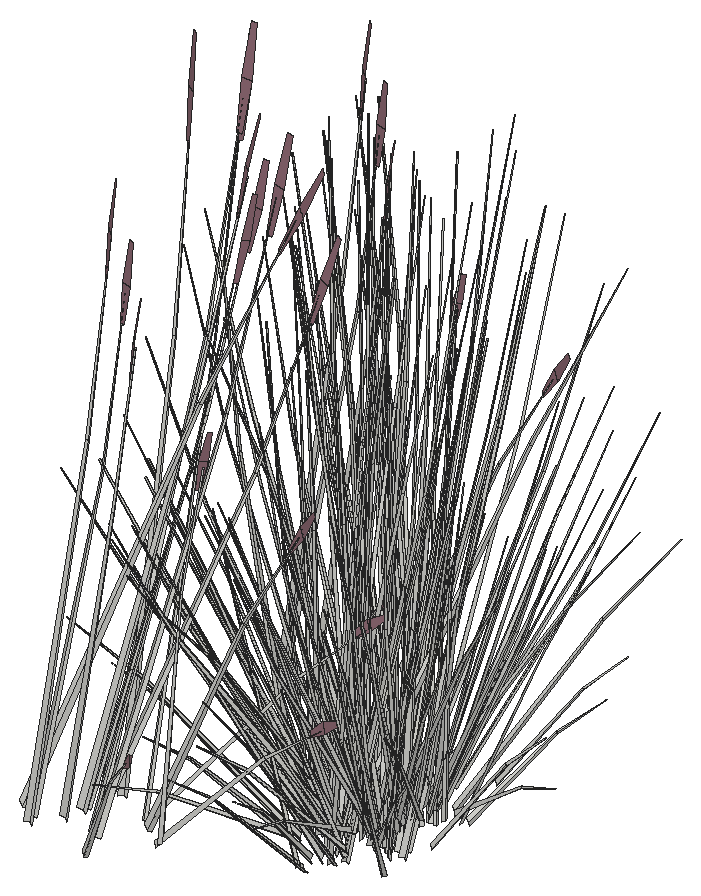
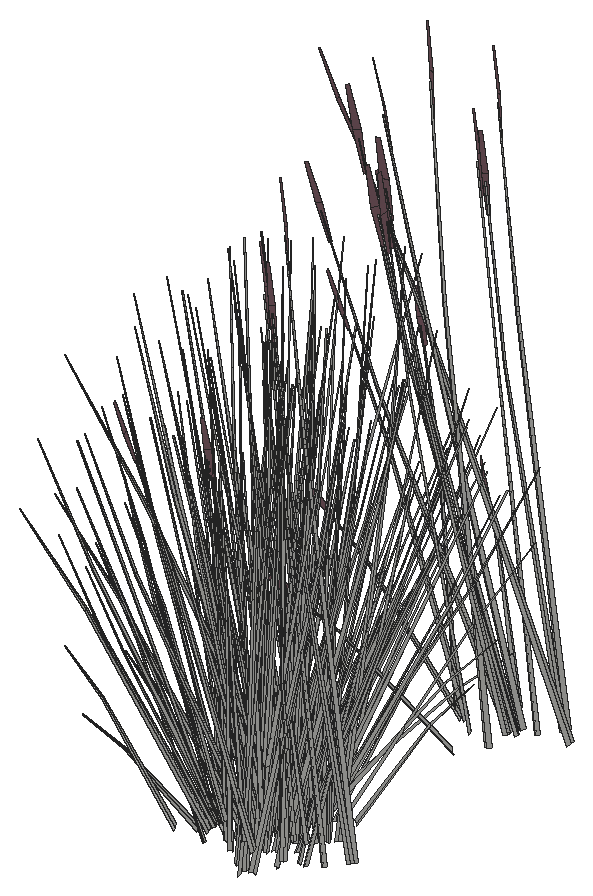
# SketchUp Ruby script. Lengths in inches.
U = 1.inch
M = Sketchup.active_model
def pt(a) = Geom::Point3d.new(a.map { |v| v * U })
def face(e, loops, mat)
  f = e.add_face(loops[0].map { |a| pt(a) })
  loops[1..].each { |l| e.add_face(l.map { |a| pt(a) }).erase! }
  f.material = f.back_material = mat if mat
  f
end
# faces: each face lists its corners as indices into pts; further lists are holes
def faces(e, pts, list, mat = nil) = list.each { |f| face(e, (f[0].is_a?(Array) ? f : [f]).map { |l| l.map { |i| pts[i] } }, mat) }
# xy, xz, yz: faces in a plane at the given z, y or x. An outline is a flat list of corners, or four numbers for a rectangle; further outlines are holes
def ring(l) = l.size == 4 ? [[l[0], l[1]], [l[2], l[1]], [l[2], l[3]], [l[0], l[3]]] : l.each_slice(2).to_a
def flat(e, list, mat, &to3) = list.each { |f| face(e, (f[0].is_a?(Array) ? f : [f]).map { |l| ring(l).map { |u, v| to3.(u, v) } }, mat) }
def xy(e, z, list, mat = nil) = flat(e, list, mat) { |x, y| [x, y, z] }
def xz(e, y, list, mat = nil) = flat(e, list, mat) { |x, z| [x, y, z] }
def yz(e, x, list, mat = nil) = flat(e, list, mat) { |y, z| [x, y, z] }
def lines(e, pts, list) = list.each { |a, b| e.add_line(pt(pts[a]), pt(pts[b])) }
# prism: a flat outline (further loops are holes) pulled along v
def prism(e, loops, v, mat = nil)
  f = face(e, loops, mat); d = Geom::Vector3d.new(v.map { |x| x * U })
  f.pushpull(f.normal.samedirection?(d) ? d.length : -d.length)
end
def box(e, o, s, mat = nil) = prism(e, [[o, [o[0] + s[0], o[1], o[2]], [o[0] + s[0], o[1] + s[1], o[2]], [o[0], o[1] + s[1], o[2]]]], [0, 0, s[2]], mat)
def at(x, y, z, deg = 0) = Geom::Transformation.translation(pt([x, y, z])) * Geom::Transformation.rotation(ORIGIN, Z_AXIS, deg.degrees)
def axes(o, x, y, z) = Geom::Transformation.new([*x, 0, *y, 0, *z, 0, *pt(o).to_a, 1])
def part(name) = M.definitions.add(name)
# library, detail: a bought-in or finely detailed component or shape, given as its bounding box
def library(name, o, s) = part(name).tap { |d| box(d.entities, o, s) }
def detail(e, o, s) = box(e.add_group.entities, o, s)
def put(e, d, t, mat = nil) = e.add_instance(d, t).tap { |i| i.material = mat if mat }
def group(e, t, mat = nil) = e.add_group.tap { |g| g.transformation = t; g.material = mat if mat }.entities
root = M.entities
M.materials.add("LightPink_Translucent").color = [144, 107, 117]
c1 = part("blade")
p = [[2.15,0.21,22],[0,0.17,0],[0.09,0.45,0],[2.18,0.31,22],[2.29,0.31,22],[0.38,0.45,0],
  [2.48,0.24,33],[2.49,0.24,33],[2.48,0.22,33]]
faces(c1.entities,p,[[0,1,2,3],[4,5,2,3],[6,3,4,7],[8,0,3,6]])
c2 = part("seeds")
p = [[0.3,-0.1,1.38],[-0.01,-0.03,1.59],[-0.01,-0.03,0.03],[0.14,-0.07,-0.07],[0.29,-0.03,3],[0.15,0.01,3.11]]
faces(c2.entities,p,[[0,1,2,3],[1,0,4,5]],"LightPink_Translucent")
c3 = part("blade with seeds")
put(c3.entities,c1,at(0,0,0))
put(c3.entities,c2,axes([2.4,0.25,30.99],[1.5799,-0.05474,1.17369],[-0.12525,1.92788,0.29478],[-0.07173,-0.02425,1.56792]))
c4 = part("blade with seeds\#1")
put(c4.entities,c1,at(0,0,0))
put(root,c3,axes([62.45,49.91,44.03],[1.14332,0.25625,-0.30978],[-0.28787,0.90242,0.30978],[0.23049,-0.10406,1.38974]))
put(root,c4,axes([73.33,39.71,40.79],[-0.89213,0.297,-0.46065],[-0.15606,-1.12475,-0.35681],[-0.23962,-0.32232,0.88141]))
put(root,c3,axes([65.59,26.18,44.67],[1.38012,0.49416,-0.29095],[-0.66454,1.04299,-0.50002],[0.04337,0.25608,1.59708]))
put(root,c4,axes([73.69,39.68,41.0625],[-0.77091,-0.6039,-0.64046],[0.54787,-1.05824,0.07729],[-0.27931,-0.36058,0.906]))
put(root,c3,axes([62.65,22.63,44.03],[1.14332,0.25625,-0.30978],[-0.28787,0.90242,0.30978],[0.23049,-0.10406,1.38974]))
put(root,c4,axes([73.97,39.18,41.11],[-0.53874,1.06944,-0.10962],[-0.78019,-0.61612,-0.60845],[-0.2712,-0.30214,0.92453]))
put(root,c3,axes([62.18,49.5,44.02],[1.14694,-0.51783,-0.49651],[0.68554,0.92854,0],[0.26122,-0.11794,1.57504]))
put(root,c3,axes([69.18,27.38,44.02],[0,1.03566,-0.49651],[-1.37109,0,0],[0,0.23588,1.57504]))
put(root,c4,axes([71.58,45.69,41.13],[0.78697,-0.17856,0.31925],[0.2078,1.02074,-0.41216],[-0.22552,0.27417,0.78863]))
put(root,c3,axes([62.38,22.22,44.02],[1.14694,-0.51783,-0.49651],[0.68554,0.92854,0],[0.26122,-0.11794,1.57504]))
put(root,c4,axes([72.98,38.81,38.91],[-0.02894,0.41302,1.28914],[-0.77632,0.42312,-0.27724],[-0.21961,-0.50739,0.55117]))
put(root,c4,axes([71.29,45.23,38.39],[-0.48852,-1.08202,-0.44759],[0.87598,-0.64674,0],[-0.11126,-0.24644,1.41987]))
put(root,c4,axes([73.73,36.55,40.82],[-0.00742,0.151,1.59908],[-0.79509,0.62706,-0.1511],[-0.26143,-0.25182,0.28298]))
put(root,c4,axes([71.56,38.33,39.07],[0.49736,0.38508,1.03545],[-0.66822,0.331,0.76078],[-0.16744,-0.31805,0.22807]))
put(root,c4,axes([74.1875,48.82,38.39],[-0.97703,0,-0.44759],[0,-1.29348,0],[-0.22253,0,1.41987]))
put(root,c4,axes([76.91,43.6,39.57],[0.39398,-0.99907,1.36359],[0.84877,0.97875,0.53923],[-0.50305,0.4384,1.14314]))
put(root,c4,axes([73.3,43.94,38.43],[-0.73437,-0.77871,-0.5621],[0.66591,-0.96736,-0.14753],[-0.18319,-0.31204,1.24074]))
put(root,c3,axes([65.33,28.59,44.18],[1.2866,-0.3514,-0.19198],[0.45209,1.01223,0.00008],[0.14202,-0.03884,1.73897]))
put(root,c4,axes([73.42,38.88,40.65],[-0.13963,-1.00636,-0.31925],[0.79822,-0.26574,0.41216],[-0.2144,-0.28839,0.78863]))
put(root,c4,axes([74.58,45.3,38.57],[-0.88038,-0.56093,-0.40331],[0.4237,-1.16553,0.1941],[-0.20294,0,1.29492]))
put(root,c4,axes([73.9,39.7,41.13],[0.13963,1.00636,0.31925],[-0.79822,0.26574,-0.41216],[-0.2144,-0.28839,0.78863]))
put(root,c4,axes([74.15,44.79,38.98],[-1.11485,0.13472,-0.26229],[-0.06741,-1.40314,-0.45076],[-0.1485,-0.24708,1.43974]))
put(root,c4,axes([74.21,48.27,38.4],[-0.60959,-0.80703,-0.27926],[0.60959,-0.80703,0.27926],[-0.19635,0,1.25283]))
put(root,c4,axes([75.32,45.44,38.98],[-0.46619,1.302,-0.26229],[-0.98396,-0.62692,-0.45076],[-0.24158,0.04092,1.43974]))
put(root,c4,axes([74.93,49.14,38.71],[0,1.44565,0],[-1.09198,0,-0.46523],[-0.24871,0,1.47583]))
put(root,c3,axes([65.35,25.58,44.21],[0.73619,0.86927,-0.44739],[-1.11511,0.61213,0.21531],[0.23824,0.10756,1.43643]))
put(root,c4,axes([71.68,44.97,38.4],[0.24175,-1.0786,-0.27926],[0.85134,0.27158,0.27926],[-0.09817,-0.21744,1.25283]))
put(root,c3,axes([63.54,51.63,44.06],[0.82544,-0.77843,-0.62353],[1.0254,0.70586,-0.16365],[0.33076,-0.19418,1.37633]))
put(root,c3,axes([63.74,24.34,44.06],[0.82544,-0.77843,-0.62353],[1.0254,0.70586,-0.16365],[0.33076,-0.19418,1.37633]))
put(root,c4,axes([73.6,39.01,40.84],[0.89921,-0.28673,0.43274],[0.15606,1.12475,0.35681],[-0.21148,-0.33149,0.89544]))
put(root,c4,axes([73.77,38.79,40.84],[0.4109,-0.79368,0.05797],[0.58514,0.46209,0.45634],[-0.18917,-0.25446,0.69585]))
put(root,c4,axes([74.68,35.98,40.82],[-0.14882,-0.16043,1.57709],[-0.91289,0.20534,-0.24942],[-0.17308,-0.40254,0.12648]))
put(root,c4,axes([74.64,48.02,38.67],[0.82143,1.07538,0.27726],[-0.81279,1.07603,-0.32897],[-0.23327,0.03755,1.48641]))
put(root,c3,axes([67.37,23.65,44.03],[0.28787,0.90242,-0.30978],[-1.14332,0.25625,0.30978],[0.23049,0.10406,1.38974]))
put(root,c3,axes([64.57,25.09,44.67],[1.23732,-0.68758,-0.29095],[0.8228,0.97154,-0.50002],[0.30528,0.09867,1.59708]))
put(root,c4,axes([75.02,44.6,38.77],[0.47355,-1.30265,0.21694],[0.98396,0.62692,0.45076],[-0.22682,0,1.44726]))
put(root,c4,axes([76.35,45.11,38.77],[-1.15773,-0.30643,-0.21121],[0.20181,-1.4529,0.4622],[-0.15988,0.25387,1.41028]))
put(root,c4,axes([74.36,45.02,39.02],[0.06031,1.25545,0.40331],[-1.00118,0.11354,-0.1941],[-0.10147,-0.22475,1.29492]))
put(root,c4,axes([75.09,48.27,38.81],[0.97703,0,0.44759],[0,1.29348,0],[-0.22253,0,1.41987]))
put(root,c4,axes([71.69,40.89,38.72],[-0.97904,-0.72283,0],[0.54599,-1.20931,-0.46523],[0.12435,-0.27543,1.47583]))
put(root,c4,axes([74.72,45.07,38.7],[1.09253,-0.50265,0.41247],[0.37991,1.43622,0.16186],[-0.20075,-0.01755,1.43206]))
put(root,c4,axes([76.07,39.14,41.11],[-0.88471,0.5817,-0.10962],[-0.43476,-1.03242,-0.60845],[-0.11673,-0.43507,0.92453]))
put(root,c4,axes([75.3125,39.1875,40.79],[-0.88873,-0.31321,-0.46065],[0.30463,-1.07385,-0.35681],[-0.08149,-0.43235,0.88141]))
put(root,c4,axes([75.88,45.21,38.57],[-0.82007,0.69452,-0.40331],[-0.57748,-1.05199,0.1941],[-0.10147,0.22475,1.29492]))
put(root,c3,axes([61.44,24.48,43.59],[-1.20625,0.41464,1.28929],[-0.38394,-1.1897,0.50096],[0.74071,0.01979,1.46642]))
put(root,c4,axes([75.5625,38.04,38.36],[0.11725,0.74462,1.27635],[-0.9333,0.11852,0.07306],[-0.14126,-0.52153,0.72629]))
put(root,c4,axes([74.73,36.68,38.61],[-0.62476,0.71677,-0.05849],[-0.57245,-0.78502,-0.26518],[-0.0403,-0.22243,0.87466]))
put(root,c4,axes([72.2,41.51,38.81],[-0.48852,1.08202,0.44759],[-0.87598,-0.64674,0],[0.11126,-0.24644,1.41987]))
put(root,c4,axes([75.58,45.32,39.02],[0.88038,0.56093,0.40331],[-0.4237,1.16553,-0.1941],[-0.20294,0,1.29492]))
put(root,c4,axes([74.82,43.26,38.5625],[-1.1305,0,0],[0,-1.44565,0],[0,0,1.61777]))
put(root,c3,axes([68.0625,49.47,43.49],[-0.18342,-0.08159,1.76342],[-0.47115,-0.9115,-0.26939],[0.31784,-0.24736,0.30037]))
put(root,c4,axes([74.1,43.95,38.7],[0.88667,0.95859,0.41247],[-0.7827,1.13884,0.16186],[-0.08849,-0.2311,1.43206]))
put(root,c3,axes([68.27,22.1875,43.49],[-0.18342,-0.08159,1.76342],[-0.47115,-0.9115,-0.26939],[0.31784,-0.24736,0.30037]))
put(root,c4,axes([72.64,45.61,38.8],[0.971,0.33398,0.15904],[-0.27478,1.22215,0.3163],[-0.00473,-0.21112,1.44604]))
put(root,c4,axes([75.63,39.39,41.0625],[-0.4315,-1.0159,-0.64046],[0.88824,-0.56616,0.07729],[-0.1009,-0.49086,0.906]))
put(root,c4,axes([73.43,46.12,38.01],[0.39117,1.13797,1.16227],[-1.12236,0.3622,0.45161],[0.01867,-0.69878,1.32195]))
put(root,c4,axes([75.69,42.9,38.65],[-0.84094,1.07538,-0.05527],[-0.84146,-1.07603,0],[-0.02937,0.03755,1.58274]))
put(root,c3,axes([67.68,23.26,44.02],[1.14694,0.51783,-0.49651],[-0.68554,0.92854,0],[0.26122,0.11794,1.57504]))
put(root,c4,axes([75.8,39.54,41.13],[-0.27256,0.96081,0.31925],[-0.79518,-0.28024,-0.41216],[-0.07291,-0.38684,0.78863]))
put(root,c3,axes([67.63,30.63,43.49],[0.08928,-0.14952,1.76342],[1.12407,-0.44035,-0.26939],[0.34078,0.22791,0.30037]))
put(root,c4,axes([73.72,43.06,38.93],[-0.87196,-0.22303,0.13053],[0.15136,-1.08968,-0.37274],[0.08953,-0.19831,1.14258]))
put(root,c4,axes([74.95,37.23,37.92],[-0.14833,0.06042,1.5897],[-0.86768,-0.41907,-0.24285],[-0.01248,-0.42273,0.27078]))
put(root,c4,axes([73.95,43.52,39.02],[-0.82007,0.69452,0.40331],[-0.57748,-1.05199,-0.1941],[0.10147,-0.22475,1.29492]))
put(root,c4,axes([75.79,44.94,38.7],[0.20585,-1.46124,0.41247],[1.16261,0.29738,0.16186],[-0.11226,0.21355,1.43206]))
put(root,c3,axes([71.23,53.15,44.26],[-0.75977,-0.66224,-0.06488],[0.83212,-0.6068,-0.29416],[0.23578,-0.04272,0.97024]))
put(root,c3,axes([66.01,25.25,44.06],[1.27479,0.1698,-0.62353],[-0.26901,1.04736,-0.16365],[0.38043,0.12691,1.37633]))
put(root,c3,axes([71.44,25.86,44.26],[-0.75977,-0.66224,-0.06488],[0.83212,-0.6068,-0.29416],[0.23578,-0.04272,0.97024]))
put(root,c4,axes([77.7,47.11,38.4],[-0.85134,0.27158,-0.27926],[-0.24175,-1.0786,0.27926],[-0.09817,0.21744,1.25283]))
put(root,c4,axes([72.28,40.23,38.39],[0.48852,-1.08202,-0.44759],[0.87598,0.64674,0],[0.11126,-0.24644,1.41987]))
put(root,c4,axes([74.01,43.17,38.98],[-0.64866,-1.16728,-0.26229],[0.91655,-0.77622,-0.45076],[0.09308,-0.288,1.43974]))
put(root,c4,axes([72.7,41.91,38.8],[0.25932,1.24233,0.15904],[-0.96507,0.30677,0.3163],[0.14061,-0.1108,1.44604]))
put(root,c4,axes([75.72,38.53,40.65],[0.27256,-0.96081,-0.31925],[0.79518,0.28024,0.41216],[-0.07291,-0.38684,0.78863]))
put(root,c4,axes([77.65,45.73,38.8],[-0.25932,-1.24233,0.15904],[0.96507,-0.30677,0.3163],[-0.14061,0.1108,1.44604]))
put(root,c4,axes([76.34,44.47,38.98],[0.64866,1.16728,-0.26229],[-0.91655,0.77622,-0.45076],[-0.09308,0.288,1.43974]))
put(root,c4,axes([75.07,42.28,38.5625],[0,-1.29348,0],[1.0115,0,0],[0,0,1.60831]))
put(root,c4,axes([72.65,40.53,38.4],[0.85134,-0.27158,-0.27926],[0.24175,1.0786,0.27926],[0.09817,-0.21744,1.25283]))
put(root,c4,axes([74.73,41.15,40.07],[0.02213,0.47954,1.54493],[-0.95907,-0.31812,0.12492],[0.05932,-0.68338,0.66044]))
put(root,c4,axes([74.55,42.7,38.72],[-0.20585,1.46124,0.44352],[-1.16261,-0.29738,0.17404],[0.11226,-0.21355,1.53985]))
put(root,c4,axes([76.05,38.67,40.84],[0.66618,-0.42462,0.05797],[0.32607,0.77431,0.45634],[-0.06434,-0.34133,0.69585]))
put(root,c4,axes([75.81,38.75,40.84],[0.89085,0.32663,0.43274],[-0.30463,1.07385,0.35681],[-0.05354,-0.4223,0.89544]))
put(root,c4,axes([76.625,44.58,38.93],[0.87196,0.22303,0.13053],[-0.15136,1.08968,-0.37274],[-0.08953,0.19831,1.14258]))
put(root,c4,axes([77.42,43.86,38.5625],[-0.84234,0.37722,0],[-0.29498,-1.07717,0],[0,0,1.39163]))
put(root,c4,axes([75.5,42.31,38.57],[0.63109,-0.80703,0],[0.63109,0.80703,0],[0,0,1.52591]))
put(root,c4,axes([75.23,40.125,38.8],[-0.71168,0.90835,0.15904],[-0.69029,-0.91538,0.3163],[0.14534,0.10032,1.44604]))
put(root,c4,axes([77.31,42.45,38.54],[-0.33151,-1.21377,-0.17307],[0.95493,-0.4265,0.00007],[-0.03664,-0.13398,1.56765]))
put(root,c4,axes([75.88,36.49,39.07],[0.1613,0.71432,1.03545],[-0.66662,-0.33623,0.76078],[0.04561,-0.37895,0.22807]))
put(root,c4,axes([74.15,41.8,38.43],[0.16018,-1.20264,-0.5621],[0.98808,0.25378,-0.14753],[0.11973,-0.3589,1.24074]))
put(root,c4,axes([77.7,42.03,38.8],[-0.971,-0.33398,0.15904],[0.27478,-1.22215,0.3163],[0.00473,0.21112,1.44604]))
put(root,c4,axes([76.64,43.16,38.8],[-0.78639,1.12892,-0.2271],[-0.88305,-0.94994,0.49699],[0.09199,0.304,1.51643]))
put(root,c4,axes([77.81,44.13,38.55],[-0.43865,1.16553,0],[-0.91144,-0.56093,0],[0,0,1.46678]))
put(root,c4,axes([74.76,42.32,39.02],[-0.88038,-0.56093,0.40331],[0.4237,-1.16553,-0.1941],[0.20294,0,1.29492]))
put(root,c4,axes([78.14,46.13,38.81],[0.48852,-1.08202,0.44759],[0.87598,0.64674,0],[-0.11126,0.24644,1.41987]))
put(root,c4,axes([75.27,42.53,38.64],[1.12994,0,-0.05082],[0,1.44565,0],[0.03551,0,1.61697]))
put(root,c4,axes([78.7,36.82,40.82],[-0.08553,0.10454,1.59908],[-0.91687,-0.22868,-0.1511],[-0.05858,-0.41178,0.28298]))
put(root,c4,axes([74.47,42.43,38.57],[0.82007,-0.69452,-0.40331],[0.57748,1.05199,0.1941],[0.10147,-0.22475,1.29492]))
put(root,c4,axes([75.25,39.375,38.81],[-0.97703,0,0.44759],[0,-1.29348,0],[0.22253,0,1.41987]))
put(root,c4,axes([77.93,37.73,40.12],[-0.82131,0.22128,-0.03148],[-0.18882,-1.04586,-0.14272],[0.05207,-0.2184,0.47074]))
put(root,c4,axes([77.91,40.44,41.11],[-0.99362,-0.0619,-0.10962],[0.02716,-1.17208,-0.60845],[0.06902,-0.45141,0.92453]))
put(root,c4,axes([74.96,41.83,38.93],[-0.28493,-1.07717,0.13053],[0.81364,-0.37722,-0.37274],[0.17907,0,1.14258]))
put(root,c4,axes([75.99,42.62,39.02],[-0.06031,-1.25545,0.40331],[1.00118,-0.11354,-0.1941],[0.10147,0.22475,1.29492]))
put(root,c4,axes([76.47,43.73,38.57],[0.06031,1.25545,-0.40331],[-1.00118,0.11354,0.1941],[0.10147,0.22475,1.29492]))
put(root,c4,axes([77.52,40.62,41.13],[-0.61172,0.65782,0.31925],[-0.57907,-0.75112,-0.41216],[0.08811,-0.38163,0.78863]))
put(root,c4,axes([76.95,37.83,38.91],[-0.2403,0.27843,1.28914],[-0.79492,-0.36227,-0.27724],[0.10768,-0.56334,0.55117]))
put(root,c3,axes([69.79,54.03,43.98],[-0.7893,0.12429,1.41583],[-0.12563,-0.9893,0.08104],[0.55282,-0.14974,0.80566]))
put(root,c4,axes([77.82,42.81,38.5625],[0.43865,-1.16553,0],[0.91144,0.56093,0],[0,0,1.57718]))
put(root,c4,axes([77.3125,39.42,40.82],[-0.01652,-0.24801,1.57709],[-0.75906,-0.68026,-0.24942],[0.1002,-0.44114,0.12648]))
put(root,c4,axes([76.42,42.59,38.93],[0.58702,-0.85413,0.13053],[0.66228,0.71246,-0.37274],[0.08953,0.19831,1.14258]))
put(root,c3,axes([70,26.74,43.98],[-0.7893,0.12429,1.41583],[-0.12563,-0.9893,0.08104],[0.55282,-0.14974,0.80566]))
put(root,c4,axes([78.79,42.34,38.55],[-0.98246,0.71382,-0.04636],[-0.54599,-1.20931,0.46523],[0.09354,0.298,1.4751]))
put(root,c3,axes([70.86,26.09,43.49],[-0.06405,-0.15723,1.76342],[0.44421,-0.91974,-0.26939],[0.4481,-0.01323,0.30037]))
put(root,c4,axes([77.43,40.38,41.0625],[0.02352,-1.1557,-0.64046],[0.99061,0.07762,0.07729],[0.10454,-0.48961,0.906]))
put(root,c4,axes([77.45,43.23,38.64],[1.12244,-0.50265,-0.0542],[0.39331,1.43622,0],[0.0392,-0.01755,1.55211]))
put(root,c4,axes([78.67,42.67,38.4],[-0.24175,1.0786,-0.27926],[-0.85134,-0.27158,0.27926],[0.09817,0.21744,1.25283]))
put(root,c4,axes([78.22,41.6875,38.81],[-0.48852,-1.08202,0.44759],[0.87598,-0.64674,0],[0.11126,0.24644,1.41987]))
put(root,c4,axes([75.98,39.07,38.56],[-0.00781,1.44494,-0.04486],[-1.09198,0,0.45022],[0.24858,0.04541,1.42752]))
put(root,c4,axes([75.42,38.5,38.72],[0,-1.44565,0],[1.09198,0,-0.46523],[0.24871,0,1.47583]))
put(root,c4,axes([75.03,42.2,38.98],[0.46619,-1.302,-0.26229],[0.98396,0.62692,-0.45076],[0.24158,-0.04092,1.43974]))
put(root,c4,axes([76.14,39.375,38.4],[0.60959,0.80703,-0.27926],[-0.60959,0.80703,0.27926],[0.19635,0,1.25283]))
put(root,c4,axes([76.2,42.85,38.98],[1.11485,-0.13472,-0.26229],[0.06741,1.40314,-0.45076],[0.1485,0.24708,1.43974]))
put(root,c4,axes([75.76,42.34,38.57],[0.88038,0.56093,-0.40331],[-0.4237,1.16553,0.1941],[0.20294,0,1.29492]))
put(root,c4,axes([77.84,39.69,40.65],[0.61172,-0.65782,-0.31925],[0.57907,0.75112,0.41216],[0.08811,-0.38163,0.78863]))
put(root,c4,axes([78.07,40.03,40.84],[0.74296,0.05822,0.05797],[-0.02037,0.87906,0.45634],[0.07774,-0.33673,0.69585]))
put(root,c4,axes([77.84,39.95,40.84],[0.64379,0.85247,0.43274],[-0.68369,0.73521,0.35681],[0.11875,-0.39995,0.89544]))
put(root,c4,axes([77.05,43.7,38.43],[0.73437,0.77871,-0.5621],[-0.66591,0.96736,-0.14753],[0.18319,0.31204,1.24074]))
put(root,c4,axes([74.06,41.97,40.61],[-0.50765,0.99901,1.24659],[-0.79039,-1.05487,0.53787],[0.47632,-0.32232,1.20495]))
put(root,c4,axes([76.16,38.82,38.39],[0.97703,0,-0.44759],[0,1.29348,0],[0.22253,0,1.41987]))
put(root,c4,axes([76.27,42.05,40.07],[-0.16834,0.42944,1.54493],[-0.70619,-0.88871,0.12492],[0.31858,-0.5539,0.66044]))
put(root,c4,axes([79.05,42.41,38.39],[0.48852,1.08202,-0.44759],[-0.87598,0.64674,0],[0.11126,0.24644,1.41987]))
put(root,c4,axes([78.58,42.66,41.13],[-0.78697,0.17856,0.31925],[-0.2078,-1.02074,-0.41216],[0.22552,-0.27417,0.78863]))
put(root,c4,axes([78.29,42.3125,38.67],[0.31757,-1.44738,0.27726],[1.13512,0.3621,-0.32897],[0.14207,0.23956,1.48641]))
put(root,c4,axes([78.1875,40.46,39.07],[-0.28093,0.65095,1.03545],[-0.28545,-0.84053,0.76078],[0.2418,-0.22671,0.22807]))
put(root,c4,axes([78.99,42.75,41.11],[-0.8363,-0.68892,-0.10962],[0.4818,-0.99769,-0.60845],[0.23628,-0.3468,0.92453]))
put(root,c4,axes([76.03,41.68,38.46],[0.89455,-0.42392,-0.62393],[0.32217,1.22114,-0.16376],[0.30292,-0.04686,1.37722]))
put(root,c4,axes([75.03,42.05,39.14],[-0.91991,0.03158,1.27354],[0.23846,-1.42935,0.53923],[0.50337,0.33806,1.20213]))
put(root,c4,axes([77.86,47.29,41.13],[-0.51441,-0.78225,0.31925],[0.58738,-0.7405,-0.41216],[0.29843,0.11267,0.78863]))
put(root,c4,axes([78.9,41.43,38.71],[0.97904,-0.72283,0],[0.54599,1.20931,-0.46523],[0.12435,0.27543,1.47583]))
put(root,c4,axes([78.33,48,40.84],[-0.04552,0.95007,0.05797],[-0.68742,-0.02605,0.45634],[0.26332,0.09941,0.69585]))
put(root,c4,axes([79.68,43.65,40.82],[-0.11829,-0.00342,1.59908],[-0.52187,-0.99076,-0.1511],[0.18628,-0.34414,0.28298]))
put(root,c4,axes([79.23,40.28,37.92],[-0.14106,-0.08423,1.5897],[-0.41543,-1.06044,-0.24285],[0.21501,-0.3215,0.27078]))
put(root,c4,axes([78.39,47.7,40.84],[-0.66663,0.82326,0.43274],[-0.57493,-0.87428,0.35681],[0.31276,0.15186,0.89544]))
put(root,c4,axes([78.58,41.93,40.79],[-0.23225,-1.14083,-0.46065],[0.87956,-0.19957,-0.35681],[0.25205,-0.30642,0.88141]))
put(root,c4,axes([78.71,45.1,41.13],[-0.75135,-0.34854,0.31925],[0.21915,-1.01686,-0.41216],[0.30251,-0.09324,0.78863]))
put(root,c4,axes([79.47,40.36,38.98],[-0.03064,0.74138,0.9471],[-0.6508,-0.48961,0.52291],[0.23122,-0.29288,0.74292]))
put(root,c4,axes([79.3,42.49,40.84],[0.62066,0.52545,0.05797],[-0.36135,0.74826,0.45634],[0.19899,-0.24191,0.69585]))
put(root,c4,axes([79.12,42.27,40.84],[0.22422,1.14989,0.43274],[-0.87956,0.19957,0.35681],[0.25922,-0.27044,0.89544]))
put(root,c4,axes([81.39,43.73,41.66],[-0.56051,-0.79893,-0.05849],[0.61388,-0.73204,-0.26518],[0.17394,-0.05154,0.87466]))
put(root,c4,axes([77.89,42.78,38.91],[-0.32388,-0.0204,1.28914],[-0.36177,-0.97496,-0.27724],[0.38765,-0.30097,0.55117]))
put(root,c4,axes([78.59,47.7,40.65],[0.51441,0.78225,-0.31925],[-0.58738,0.7405,0.41216],[0.29843,0.11267,0.78863]))
put(root,c4,axes([79.39,45.41,40.84],[0.33205,0.8519,0.05797],[-0.60551,0.41697,0.45634],[0.26692,-0.08227,0.69585]))
put(root,c4,axes([78,47.79,41.44],[0.04841,-1.27062,-0.12168],[0.91657,0.03473,-0.67538],[0.353,0.08826,1.02623]))
put(root,c4,axes([79.32,45.11,41.14],[-0.25543,1.1392,0.48034],[-0.83975,-0.38955,0.39606],[0.33023,-0.06846,0.99394]))
put(root,c4,axes([79.02,45.4375,41.11],[-0.45489,-1.13134,-0.10962],[0.80735,-0.55596,-0.60845],[0.34022,-0.14927,0.92453]))
put(root,c4,axes([80.59,47.2,39.07],[-0.58095,0.02992,1.03545],[0.41436,-0.74764,0.76078],[0.2769,0.14704,0.22807]))
put(root,c4,axes([79.2,45.23,37.92],[-0.05317,-0.18711,1.5897],[0.29263,-1.12549,-0.24285],[0.32981,-0.03291,0.27078]))
put(root,c4,axes([78.35,46.92,41.09],[0.65648,-0.82762,-0.51132],[0.57493,0.87428,-0.39606],[0.33354,0.12593,0.97836]))
put(root,c4,axes([77.25,43.82,40.07],[-0.31369,0.26428,1.54493],[-0.26409,-1.22118,0.12492],[0.49247,-0.276,0.66044]))
put(root,c4,axes([78.98,44.47,40.79],[0.24493,-1.13649,-0.46065],[0.83975,0.38955,-0.35681],[0.33809,-0.10421,0.88141]))
put(root,c4,axes([79.33,47.82,39.12],[-0.17302,-1.05027,0.05866],[0.69705,-0.24145,-0.77802],[0.35285,0.06658,0.69739]))
put(root,c4,axes([79.5,44.99,40.65],[0.75135,0.34854,-0.31925],[-0.21915,1.01686,0.41216],[0.30251,-0.09324,0.78863]))
put(root,c4,axes([78.05,47.18,41.39],[0.90375,0.03008,-0.71091],[-0.0607,1.26677,0.08579],[0.38287,0.13368,1.00565]))
put(root,c4,axes([77.41,45.98,40.07],[-0.375,0.0283,1.54493],[0.24877,-1.22643,0.12492],[0.53441,0.07586,0.66044]))
put(root,c4,axes([80.42,50.49,40.82],[-0.05899,-0.13116,1.59908],[0.39237,-1.08407,-0.1511],[0.32669,0.02548,0.28298]))
put(root,c4,axes([78.82,44.88,41.0625],[0.79444,-0.5518,-0.64046],[0.44274,1.13586,0.07729],[0.38385,-0.12903,0.906]))
put(root,c4,axes([80.83,45.71,40.82],[0.15733,-0.14655,1.57709],[0.06181,-1.18266,-0.24942],[0.34698,-0.11893,0.12648]))
put(root,c4,axes([79.32,47.6,39.61],[-0.50438,-0.0254,1.3914],[0.26641,-1.14247,0.19228],[0.53755,0.09899,0.65702]))
